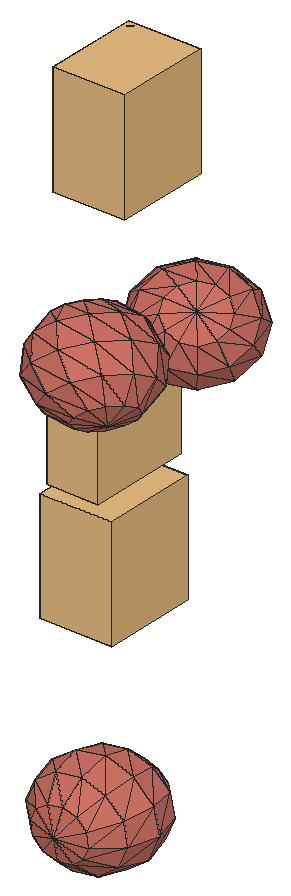
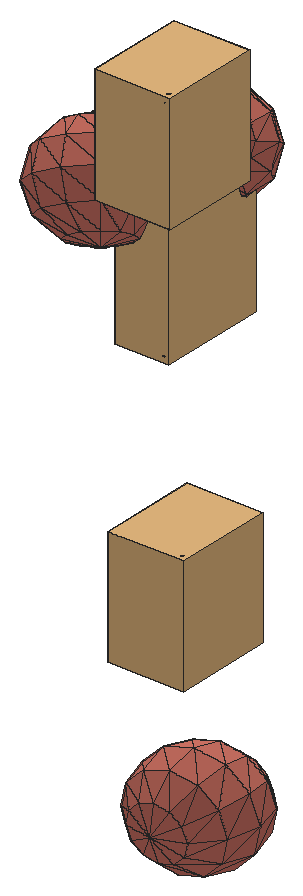
# SketchUp Ruby script. Lengths in inches.
U = 1.inch
M = Sketchup.active_model
def pt(a) = Geom::Point3d.new(a.map { |v| v * U })
def face(e, loops, mat)
  f = e.add_face(loops[0].map { |a| pt(a) })
  loops[1..].each { |l| e.add_face(l.map { |a| pt(a) }).erase! }
  f.material = f.back_material = mat if mat
  f
end
# faces: each face lists its corners as indices into pts; further lists are holes
def faces(e, pts, list, mat = nil) = list.each { |f| face(e, (f[0].is_a?(Array) ? f : [f]).map { |l| l.map { |i| pts[i] } }, mat) }
# xy, xz, yz: faces in a plane at the given z, y or x. An outline is a flat list of corners, or four numbers for a rectangle; further outlines are holes
def ring(l) = l.size == 4 ? [[l[0], l[1]], [l[2], l[1]], [l[2], l[3]], [l[0], l[3]]] : l.each_slice(2).to_a
def flat(e, list, mat, &to3) = list.each { |f| face(e, (f[0].is_a?(Array) ? f : [f]).map { |l| ring(l).map { |u, v| to3.(u, v) } }, mat) }
def xy(e, z, list, mat = nil) = flat(e, list, mat) { |x, y| [x, y, z] }
def xz(e, y, list, mat = nil) = flat(e, list, mat) { |x, z| [x, y, z] }
def yz(e, x, list, mat = nil) = flat(e, list, mat) { |y, z| [x, y, z] }
def lines(e, pts, list) = list.each { |a, b| e.add_line(pt(pts[a]), pt(pts[b])) }
# prism: a flat outline (further loops are holes) pulled along v
def prism(e, loops, v, mat = nil)
  f = face(e, loops, mat); d = Geom::Vector3d.new(v.map { |x| x * U })
  f.pushpull(f.normal.samedirection?(d) ? d.length : -d.length)
end
def box(e, o, s, mat = nil) = prism(e, [[o, [o[0] + s[0], o[1], o[2]], [o[0] + s[0], o[1] + s[1], o[2]], [o[0], o[1] + s[1], o[2]]]], [0, 0, s[2]], mat)
def at(x, y, z, deg = 0) = Geom::Transformation.translation(pt([x, y, z])) * Geom::Transformation.rotation(ORIGIN, Z_AXIS, deg.degrees)
def axes(o, x, y, z) = Geom::Transformation.new([*x, 0, *y, 0, *z, 0, *pt(o).to_a, 1])
def part(name) = M.definitions.add(name)
# library, detail: a bought-in or finely detailed component or shape, given as its bounding box
def library(name, o, s) = part(name).tap { |d| box(d.entities, o, s) }
def detail(e, o, s) = box(e.add_group.entities, o, s)
def put(e, d, t, mat = nil) = e.add_instance(d, t).tap { |i| i.material = mat if mat }
def group(e, t, mat = nil) = e.add_group.tap { |g| g.transformation = t; g.material = mat if mat }.entities
root = M.entities
M.materials.add("green").color = [174, 139, 102]
M.materials.add("vio").color = [206, 114, 100]
c1 = library("3DGeom~144_Defintion",[-424.75,-500,-323.76],[849.5,1000,647.52])
c2 = part("3DGeom~145_Defintion")
p = [[-419.66,479.4,-302.56],[-386.2,481.32,-323.76],[-405.55,478.95,-317.48],[-419.66,479.4,-302.56],[-366.78,485.875,-319.73],[-386.2,481.32,-323.76],
  [-419.66,479.4,-302.56],[-352.51,491.39,-306.47],[-366.78,485.875,-319.73],[-419.66,479.4,-302.56],[-347.21,496.4,-287.52],[-352.51,491.39,-306.47],
  [-419.66,479.4,-302.56],[-424.75,482.55,-283.01],[-419.44,487.56,-264.0625],[-419.66,479.4,-302.56],[-366.41,500,-253.05],[-352.3,499.55,-267.97],
  [-419.66,479.4,-302.56],[-352.3,499.55,-267.97],[-347.21,496.4,-287.52],[-419.66,479.4,-302.56],[-405.17,493.08,-250.79],[-385.76,497.63,-246.76],
  [-419.66,479.4,-302.56],[-385.76,497.63,-246.76],[-366.41,500,-253.05],[-419.66,479.4,-302.56],[-419.44,487.56,-264.0625],[-405.17,493.08,-250.79],
  [368.25,-500,278.25],[381.22,-498.52,262.42],[397.44,-490.86,253.62],[422.57,-466.35,264.06],[368.25,-500,278.25],[397.44,-490.86,253.62],
  [422.57,-466.35,264.06],[397.44,-490.86,253.62],[412.58,-479.09,254.22],[418.52,-450.97,299.13],[368.25,-500,278.25],[422.57,-466.35,264.06],
  [422.57,-466.35,264.06],[424.75,-456.06,280.5],[368.25,-500,278.25],[364.2,-484.62,313.32],[362.02,-494.91,296.88],[364.2,-484.62,313.32],
  [368.25,-500,278.25],[389.33,-460.11,323.76],[389.33,-460.11,323.76],[368.25,-500,278.25],[389.33,-460.11,323.76],[405.55,-452.45,314.97],
  [364.2,-484.62,313.32],[389.33,-460.11,323.76],[374.19,-471.88,323.16]]
faces(c2.entities,p,[[0,1,2],[3,4,5],[6,7,8],[9,10,11],[12,13,14],[15,16,17],[18,19,20],[21,22,23],
  [24,25,26],[27,28,29],[30,31,32],[33,34,35],[36,37,38],[39,40,41],[39,42,43],[44,45,46],
  [47,48,49],[50,51,39],[52,39,53],[54,55,56]],"green")
c3 = library("3DGeom~140_Defintion",[-424.75,-500,-323.76],[849.5,1000,647.52])
c4 = part("3DGeom~141_Defintion")
p = [[-419.66,479.4,-302.56],[-386.2,481.32,-323.76],[-405.55,478.95,-317.48],[-419.66,479.4,-302.56],[-366.78,485.875,-319.73],[-386.2,481.32,-323.76],
  [-419.66,479.4,-302.56],[-352.51,491.39,-306.47],[-366.78,485.875,-319.73],[-419.66,479.4,-302.56],[-347.21,496.4,-287.52],[-352.51,491.39,-306.47],
  [-419.66,479.4,-302.56],[-424.75,482.55,-283.01],[-419.44,487.56,-264.0625],[-419.66,479.4,-302.56],[-366.41,500,-253.05],[-352.3,499.55,-267.97],
  [-419.66,479.4,-302.56],[-352.3,499.55,-267.97],[-347.21,496.4,-287.52],[-419.66,479.4,-302.56],[-405.17,493.08,-250.79],[-385.76,497.63,-246.76],
  [-419.66,479.4,-302.56],[-385.76,497.63,-246.76],[-366.41,500,-253.05],[-419.66,479.4,-302.56],[-419.44,487.56,-264.0625],[-405.17,493.08,-250.79],
  [368.25,-500,278.25],[381.22,-498.52,262.42],[397.44,-490.86,253.62],[422.57,-466.35,264.06],[368.25,-500,278.25],[397.44,-490.86,253.62],
  [422.57,-466.35,264.06],[397.44,-490.86,253.62],[412.58,-479.09,254.22],[418.52,-450.97,299.13],[368.25,-500,278.25],[422.57,-466.35,264.06],
  [422.57,-466.35,264.06],[424.75,-456.06,280.5],[368.25,-500,278.25],[364.2,-484.62,313.32],[362.02,-494.91,296.88],[364.2,-484.62,313.32],
  [368.25,-500,278.25],[389.33,-460.11,323.76],[389.33,-460.11,323.76],[368.25,-500,278.25],[389.33,-460.11,323.76],[405.55,-452.45,314.97],
  [364.2,-484.62,313.32],[389.33,-460.11,323.76],[374.19,-471.88,323.16]]
faces(c4.entities,p,[[0,1,2],[3,4,5],[6,7,8],[9,10,11],[12,13,14],[15,16,17],[18,19,20],[21,22,23],
  [24,25,26],[27,28,29],[30,31,32],[33,34,35],[36,37,38],[39,40,41],[39,42,43],[44,45,46],
  [47,48,49],[50,51,39],[52,39,53],[54,55,56]],"green")
c5 = part("3DGeom~230_Defintion")
p = [[-248.9,29.76,-432.23],[1.27,34.79,-498.32],[1.59,-181.375,-452.05],[251.38,-156.7,-390.8125],[251.1,30.51,-430.88],[-249.48,208.89,-356.66],
  [0.6,241.64,-411.0625],[-249.48,208.89,-356.66],[-248.62,-157.45,-392.16],[1.49,-348.94,-284.65],[251.29,-301.82,-245.84],[-248.62,-157.45,-392.16],
  [-432.38,16.75,-250.32],[-248.62,-157.45,-392.16],[-432.71,120.17,-206.7],[-248.9,29.76,-432.23],[-432.38,16.75,-250.32],[-249.48,208.89,-356.66],
  [-248.9,29.76,-432.23],[433.81,-90.04,-224.86],[433.65,18.05,-247.99],[433.81,-90.04,-224.86],[250.52,209.64,-355.32],[433.65,18.05,-247.99],
  [251.1,30.51,-430.88],[250.52,209.64,-355.32],[-250.19,331.95,-185.71],[-249.48,208.89,-356.66],[-0.22,383.74,-213.67],[250.52,209.64,-355.32],
  [0.6,241.64,-411.0625],[-250.19,331.95,-185.71],[-0.22,383.74,-213.67],[-248.62,-157.45,-392.16],[-248.71,-302.57,-247.1875],[-432.22,-91.34,-227.19],
  [-248.62,-157.45,-392.16],[-248.71,-302.57,-247.1875],[-432.38,16.75,-250.32],[-248.62,-157.45,-392.16],[-432.22,-91.34,-227.19],[251.38,-156.7,-390.8125],
  [433.76,-173.82,-141.16],[251.29,-301.82,-245.84],[251.38,-156.7,-390.8125],[433.81,-90.04,-224.86],[-433.125,191.22,-108],[-250.19,331.95,-185.71],
  [250.52,209.64,-355.32],[433.31,121.47,-204.37],[433.65,18.05,-247.99],[249.81,332.7,-184.37],[250.52,209.64,-355.32],[-0.22,383.74,-213.67],
  [249.81,332.7,-184.37],[250.52,209.64,-355.32],[-248.71,-302.57,-247.1875],[1.49,-348.94,-284.65],[0.99,-423.01,-40.98],[1.49,-348.94,-284.65],
  [250.86,-365.97,-34.82],[1.49,-348.94,-284.65],[251.29,-301.82,-245.84],[-500,-0.75,-1.35],[433.65,18.05,-247.99],[500,0.75,1.35],
  [433.65,18.05,-247.99],[-248.71,-302.57,-247.1875],[-249.14,-366.71,-36.17],[-432.27,-175.12,-143.49],[-249.14,-366.71,-36.17],[251.29,-301.82,-245.84],
  [433.51,-210.86,-19.33],[250.86,-365.97,-34.82],[251.29,-301.82,-245.84],[-250.86,365.97,34.82],[-0.22,383.74,-213.67],[-250.19,331.95,-185.71],
  [-0.99,423.01,40.98],[-0.22,383.74,-213.67],[-250.86,365.97,34.82],[-0.22,383.74,-213.67],[432.9,192.52,-105.67],[249.81,332.7,-184.37],
  [-433.51,210.86,19.33],[-250.86,365.97,34.82],[249.14,366.71,36.17],[249.81,332.7,-184.37],[249.14,366.71,36.17],[-432.52,-212.16,-21.66],
  [432.52,212.16,21.66],[249.14,366.71,36.17],[-249.14,-366.71,-36.17],[0.22,-383.74,213.67],[250.19,-331.95,185.71],[250.19,-331.95,185.71],
  [-249.14,-366.71,-36.17],[-249.81,-332.7,184.37],[-249.81,-332.7,184.37],[250.86,-365.97,-34.82],[433.125,-191.22,108],[250.19,-331.95,185.71],
  [250.86,-365.97,-34.82],[-432.9,-192.52,105.67],[-433.3125,-121.47,204.37],[-433.65,-18.05,247.99],[-433.81,90.04,224.86],[-433.76,173.82,141.16],
  [432.71,-120.17,206.7],[432.38,-16.75,250.32],[432.22,91.34,227.19],[432.38,-16.75,250.32],[432.27,175.12,143.49],[248.71,302.57,247.1875],
  [248.71,302.57,247.1875],[249.14,366.71,36.17],[-251.29,301.82,245.84],[-251.29,301.82,245.84],[-250.86,365.97,34.82],[-1.49,348.94,284.65],
  [248.71,302.57,247.1875],[-251.29,301.82,245.84],[-250.52,-209.64,355.32],[250.19,-331.95,185.71],[248.62,157.45,392.16],[248.62,157.45,392.16],
  [248.71,302.57,247.1875],[-249.81,-332.7,184.37],[-0.6,-241.64,411.0625],[-249.81,-332.7,184.37],[-0.6,-241.64,411.0625],[-250.52,-209.64,355.32],
  [0.22,-383.74,213.67],[250.19,-331.95,185.71],[249.48,-208.89,356.66],[250.19,-331.95,185.71],[249.48,-208.89,356.66],[-251.1,-30.51,430.88],
  [-251.1,-30.51,430.88],[249.48,-208.89,356.66],[432.38,-16.75,250.32],[0.22,-383.74,213.67],[-0.6,-241.64,411.0625],[-433.65,-18.05,247.99],
  [-251.38,156.7,390.8125],[-433.81,90.04,224.86],[-251.38,156.7,390.8125],[248.9,-29.76,432.23],[432.22,91.34,227.19],[248.62,157.45,392.16],
  [432.38,-16.75,250.32],[432.22,91.34,227.19],[-251.38,156.7,390.8125],[-1.49,348.94,284.65],[-251.29,301.82,245.84],[-1.59,181.375,452.05],
  [248.71,302.57,247.1875],[248.71,302.57,247.1875],[-1.49,348.94,284.65],[-433.65,-18.05,247.99],[-251.1,-30.51,430.88],[-251.38,156.7,390.8125],
  [249.48,-208.89,356.66],[432.38,-16.75,250.32],[248.9,-29.76,432.23],[-251.38,156.7,390.8125],[-1.49,348.94,284.65],[-250.52,-209.64,355.32],
  [-1.27,-34.79,498.32],[-250.52,-209.64,355.32],[-251.38,156.7,390.8125]]
faces(c5.entities,p,[[0,1,2],[1,3,2],[1,4,3],[5,1,0],[6,4,1],[7,6,1],[8,2,9],[2,10,9],
  [2,3,10],[0,2,11],[12,0,13],[14,15,16],[14,17,18],[4,19,3],[4,20,21],[22,23,24],
  [6,25,4],[26,6,27],[28,29,30],[31,32,6],[33,9,34],[35,36,37],[38,39,40],[41,42,43],
  [44,45,42],[46,17,14],[46,47,17],[48,49,50],[51,49,52],[53,54,55],[56,57,58],[59,60,58],
  [61,62,60],[16,35,63],[14,16,63],[45,64,65],[66,49,65],[67,58,68],[69,37,70],[35,37,69],
  [71,72,73],[74,42,72],[35,69,63],[42,45,65],[75,76,77],[78,54,79],[80,78,81],[46,14,63],
  [49,82,65],[83,82,49],[84,47,46],[84,85,47],[86,82,87],[78,88,54],[69,70,89],[69,89,63],
  [72,42,65],[84,46,63],[82,90,65],[91,90,82],[92,58,93],[58,94,93],[58,60,95],[96,93,97],
  [89,70,98],[99,100,101],[102,72,100],[89,98,103],[89,103,63],[100,72,65],[103,104,63],[104,105,63],
  [105,106,63],[107,84,63],[106,107,63],[108,100,65],[109,108,65],[110,111,65],[112,110,65],[90,112,65],
  [107,85,84],[113,112,90],[114,90,115],[107,116,85],[117,78,118],[119,120,88],[119,88,78],[121,119,78],
  [103,98,122],[103,122,104],[123,100,108],[106,116,107],[124,110,112],[125,112,126],[127,93,128],[129,130,131],
  [132,133,134],[135,108,136],[104,122,137],[104,138,105],[139,108,140],[141,134,142],[143,144,145],[106,146,116],
  [147,148,149],[147,150,151],[152,153,154],[155,149,156],[155,157,158],[159,160,161],[162,163,164],[165,155,166],
  [167,142,168],[169,168,160],[142,134,147],[160,155,170],[168,149,155],[168,147,149],[142,147,168],[160,168,155]],"vio")
c6 = library("3DGeom~152_Defintion",[-440.97,-500,-219.08],[881.94,1000,438.17])
c7 = part("3DGeom~153_Defintion")
p = [[-380.69,-485.53,-210.54],[-411.26,-467,-218.1875],[-394.16,-475.51,-219.08],[-380.69,-485.53,-210.54],[-434.74,-476.74,-157.14],[-411.26,-467,-218.1875],
  [-438.29,-462.61,-191.49],[-411.26,-467,-218.1875],[-438.29,-462.61,-191.49],[-427.41,-462.28,-208.09],[-377.14,-499.67,-176.1875],[-434.74,-476.74,-157.14],
  [-380.69,-485.53,-210.54],[-377.14,-499.67,-176.1875],[-380.69,-485.53,-210.54],[-374.46,-494.375,-194.84],[-434.74,-476.74,-157.14],[-440.97,-467.9,-172.84],
  [-438.29,-462.61,-191.49],[-404.17,-495.28,-149.49],[-377.14,-499.67,-176.1875],[-388.02,-500,-159.59],[-404.17,-495.28,-149.49],[-434.74,-476.74,-157.14],
  [-404.17,-495.28,-149.49],[-421.27,-486.76,-148.59],[402.51,492.03,208.37],[431.04,458.58,149.1],[419.28,470.25,140.95],[402.51,492.03,208.37],
  [419.28,470.25,140.95],[406.85,483.28,142.92],[402.51,492.03,208.37],[406.85,483.28,142.92],[397.08,494.16,154.49],[402.51,492.03,208.37],
  [438.98,451.39,165.19],[431.04,458.58,149.1],[402.51,492.03,208.37],[397.08,494.16,154.49],[392.58,500,172.55],[402.51,492.03,208.37],
  [440.97,450.61,184.92],[438.98,451.39,165.19],[402.51,492.03,208.37],[392.58,500,172.55],[394.57,499.22,192.28],[402.51,492.03,208.37],
  [436.48,456.44,202.98],[440.97,450.61,184.92],[402.51,492.03,208.37],[426.7,467.33,214.55],[402.51,492.03,208.37],[414.27,480.36,216.53],
  [426.7,467.33,214.55]]
faces(c7.entities,p,[[0,1,2],[3,4,5],[5,4,6],[7,8,9],[10,11,12],[13,14,15],[16,17,18],[19,20,21],
  [22,11,10],[23,24,25],[26,27,28],[29,30,31],[32,33,34],[35,36,37],[38,39,40],[41,42,43],
  [44,45,46],[47,48,49],[50,51,48],[52,53,54]],"green")
c8 = part("3DGeom~238_Defintion")
p = [[47.04,-55.62,-493.71],[-13.56,-317.59,-331.8],[-140.27,-151.99,-445.55],[202.73,-206.32,-387.4],[187.3,88.625,-451.96],[-121.25,109.98,-467.72],
  [-40.27,193.26,-443.62],[-229.4,54.34,-439.92],[-257.06,246.11,-316.41],[364.69,-39.76,-339.2],[242.94,242.1,-331.5],[-8.15,281.87,-374.07],
  [-226.21,-343.77,-187.29],[-324.43,-174.66,-320.41],[-335.72,41.26,-367.67],[202.73,-206.32,-387.4],[116.79,-398.1,-129.14],[-13.56,-317.59,-331.8],
  [202.73,-206.32,-387.4],[304.09,-301.73,-177.3],[364.69,-39.76,-339.2],[304.09,-301.73,-177.3],[202.73,-206.32,-387.4],[-33.49,352.06,-277.72],
  [242.94,242.1,-331.5],[-8.15,281.87,-374.07],[-33.49,352.06,-277.72],[-335.72,41.26,-367.67],[-324.43,-174.66,-320.41],[-456.1,-117.55,-151.8],
  [-335.72,41.26,-367.67],[-411.74,74.22,-270.32],[-335.72,41.26,-367.67],[-257.06,246.11,-316.41],[364.69,-39.76,-339.2],[444.36,-157.49,-135.55],
  [304.09,-301.73,-177.3],[428.9375,137.45,-200.11],[364.69,-39.76,-339.2],[428.9375,137.45,-200.11],[-13.56,-317.59,-331.8],[-67.38,-420.77,-4],
  [-226.21,-343.77,-187.29],[-13.56,-317.59,-331.8],[199.05,363.67,-164.61],[428.9375,137.45,-200.11],[242.94,242.1,-331.5],[-33.49,352.06,-277.72],
  [199.05,363.67,-164.61],[242.94,242.1,-331.5],[-324.43,-174.66,-320.41],[-226.21,-343.77,-187.29],[-378.25,-277.83,7.4],[-324.43,-174.66,-320.41],
  [-437.09,144.42,-173.96],[-257.06,246.11,-316.41],[-404.96,233.02,-104.42],[-257.06,246.11,-316.41],[-323.98,316.3,-80.32],[-257.06,246.11,-316.41],
  [-323.98,316.3,-80.32],[-215.84,371.9375,-108.12],[-257.06,246.11,-316.41],[-109.51,385.02,-180.37],[-33.49,352.06,-277.72],[-257.06,246.11,-316.41],
  [-257.06,246.11,-316.41],[-33.49,352.06,-277.72],[-500,4.02,15.09],[428.9375,137.45,-200.11],[500,-4.02,-15.09],[378.25,277.83,-7.4],
  [428.9375,137.45,-200.11],[199.05,363.67,-164.61],[428.9375,137.45,-200.11],[-226.21,-343.77,-187.29],[-199.05,-363.67,164.61],[-226.21,-343.77,-187.29],
  [-199.05,-363.67,164.61],[-378.25,-277.83,7.4],[67.38,420.77,4],[215.84,-371.9375,108.12],[323.98,-316.3,80.32],[323.98,-316.3,80.32],
  [304.09,-301.73,-177.3],[-444.36,157.49,135.55],[378.25,277.83,-7.4],[-428.9375,-137.45,200.11],[404.96,-233.02,104.42],[323.98,-316.3,80.32],
  [109.51,-385.02,180.37],[-116.78,398.1,129.14],[-304.09,301.73,177.3],[-304.09,301.73,177.3],[-323.98,316.3,-80.32],[-304.09,301.73,177.3],
  [437.09,-144.42,173.96],[456.1,117.55,151.8],[226.21,343.77,187.29],[226.21,343.77,187.29],[378.25,277.83,-7.4],[33.49,-352.06,277.72],
  [-199.05,-363.67,164.61],[-199.05,-363.67,164.61],[-242.94,-242.09,331.5],[-242.94,-242.09,331.5],[-364.69,39.76,339.2],[257.06,-246.11,316.41],
  [323.98,-316.3,80.32],[257.06,-246.11,316.41],[257.06,-246.11,316.41],[13.56,317.59,331.8],[-202.73,206.32,387.4],[-202.73,206.32,387.4],
  [-304.09,301.73,177.3],[411.74,-74.22,270.32],[324.43,174.66,320.41],[226.21,343.77,187.29],[-199.05,-363.67,164.61],[8.15,-281.87,374.07],
  [-242.94,-242.09,331.5],[-199.05,-363.67,164.61],[8.15,-281.87,374.07],[257.06,-246.11,316.41],[-202.73,206.32,387.4],[13.56,317.59,331.8],
  [324.43,174.66,320.41],[226.21,343.77,187.29],[-428.9375,-137.45,200.11],[-242.94,-242.09,331.5],[-187.3,-88.625,451.96],[-428.9375,-137.45,200.11],
  [-364.69,39.76,339.2],[335.72,-41.26,367.67],[257.06,-246.11,316.41],[8.15,-281.87,374.07],[33.49,-352.06,277.72],[257.06,-246.11,316.41],
  [40.27,-193.26,443.62],[257.06,-246.11,316.41],[121.25,-109.98,467.72],[257.06,-246.11,316.41],[229.4,-54.34,439.92],[257.06,-246.11,316.41],
  [335.72,-41.26,367.67],[257.06,-246.11,316.41],[140.27,151.99,445.55],[335.72,-41.26,367.67],[324.43,174.66,320.41],[13.56,317.59,331.8],
  [324.43,174.66,320.41],[-202.73,206.32,387.4],[13.56,317.59,331.8],[-364.69,39.76,339.2],[-47.04,55.62,493.71],[-364.69,39.76,339.2],
  [-202.73,206.32,387.4],[335.72,-41.26,367.67],[-202.73,206.32,387.4]]
faces(c8.entities,p,[[0,1,2],[0,3,1],[4,3,0],[5,0,2],[6,0,5],[6,4,0],[5,2,7],[5,7,8],
  [6,5,8],[4,9,3],[10,9,4],[11,4,6],[11,10,4],[2,12,13],[2,1,12],[7,2,13],
  [11,6,8],[7,13,14],[7,14,8],[15,16,17],[18,19,16],[20,21,22],[23,24,25],[26,11,8],
  [27,28,29],[30,29,31],[32,31,33],[34,35,36],[37,35,38],[10,39,9],[40,41,42],[43,16,41],
  [44,45,46],[47,48,49],[50,51,52],[53,52,29],[31,54,55],[54,56,57],[56,58,59],[60,61,62],
  [63,64,65],[61,63,66],[63,48,67],[31,29,68],[31,68,54],[69,70,35],[71,70,72],[73,71,74],
  [75,41,76],[77,78,79],[63,80,48],[61,80,63],[19,81,16],[19,82,81],[35,83,84],[54,68,85],
  [54,85,56],[80,86,48],[29,52,87],[29,87,68],[35,88,89],[70,88,35],[16,90,41],[16,81,90],
  [60,91,61],[61,91,80],[56,85,92],[56,93,94],[60,95,91],[70,96,88],[97,96,70],[71,97,70],
  [98,97,71],[80,99,100],[41,101,102],[41,90,101],[91,99,80],[52,103,104],[52,105,87],[68,87,106],
  [68,106,85],[81,82,107],[108,88,109],[88,96,110],[90,81,107],[95,111,91],[91,111,99],[85,106,112],
  [85,113,114],[97,115,96],[116,115,97],[117,116,97],[118,119,120],[121,101,122],[96,115,123],[95,124,111],
  [101,90,107],[125,126,127],[128,129,130],[131,130,132],[115,133,134],[116,133,115],[135,136,137],[138,135,139],
  [140,138,141],[142,140,143],[144,142,145],[146,147,148],[149,146,150],[129,135,138],[129,138,130],[151,146,152],
  [153,130,154],[155,154,156],[146,142,157],[158,154,146],[154,140,142],[154,142,146],[130,138,140],[130,140,154]],"vio")
c9 = part("3DGeom~206_Defintion")
p = [[-12.5,-12.78,-500],[-167.87,-176.1875,-423.23],[-275,-119.8,-393.5],[139.12,-146.19,-448.74],[321.29,0,-383.61],[-198.05,84.89,-448.51],
  [146.22,154.06,-442.79],[216.18,-279.61,-308.47],[-80.33,-253.22,-393.64],[410.28,-154.06,-221.63],[410.28,-154.06,-221.63],[-373.01,-99.16,-312.41],
  [-373.01,-99.16,-312.41],[-367.81,120.64,-308.0625],[-68.03,266.84,-383.34],[-367.81,120.64,-308.0625],[-68.03,266.84,-383.34],[417.375,146.19,-215.68],
  [417.375,146.19,-215.68],[265.76,279.61,-266.94],[265.76,279.61,-266.94],[-68.03,266.84,-383.34],[-278.26,-292.39,-233.06],[-278.26,-292.39,-233.06],
  [-35.84,-330.25,-312.65],[-278.26,-292.39,-233.06],[-373.01,-99.16,-312.41],[-275,-119.8,-393.5],[-278.26,-292.39,-233.06],[494.4375,12.78,-75.41],
  [410.28,-154.06,-221.63],[321.29,0,-383.61],[321.29,0,-383.61],[417.375,146.19,-215.68],[-68.03,266.84,-383.34],[-367.81,120.64,-308.0625],
  [-264.06,308.11,-221.16],[80.21,377.28,-215.45],[-68.03,266.84,-383.34],[-264.06,308.11,-221.16],[265.76,279.61,-266.94],[-68.03,266.84,-383.34],
  [80.21,377.28,-215.45],[-35.84,-330.25,-312.65],[-46.32,-386.64,-201.97],[-278.26,-292.39,-233.06],[198.04,-377.28,-116.76],[-35.84,-330.25,-312.65],
  [198.04,-377.28,-116.76],[-35.84,-330.25,-312.65],[216.18,-279.61,-308.47],[-435.64,-119.8,-201.7],[-278.26,-292.39,-233.06],[-367.81,120.64,-308.0625],
  [389.33,-266.84,-0.27],[198.04,-377.28,-116.76],[216.18,-279.61,-308.47],[216.18,-279.61,-308.47],[-476.3,84.89,-116.29],[-264.06,308.11,-221.16],
  [401.625,253.22,10.03],[265.76,279.61,-266.94],[265.76,279.61,-266.94],[314.09,330.25,-19.5625],[314.09,330.25,-19.5625],[265.76,279.61,-266.94],
  [-108.95,-407.27,-91.25],[-206.96,-386.64,-10.17],[-314.09,-330.25,19.5625],[-314.09,-330.25,19.5625],[-401.625,-253.22,-10.03],[-278.26,-292.39,-233.06],
  [-446.12,-176.1875,-91.02],[-278.26,-292.39,-233.06],[-278.26,-292.39,-233.06],[476.3,-84.89,116.29],[-264.06,308.11,-221.16],[-389.33,266.84,0.27],
  [-89.55,413.03,-75],[-389.33,266.84,0.27],[446.12,176.1875,91.02],[206.96,386.64,10.17],[89.55,-413.03,75],[198.04,-377.28,-116.76],
  [264.06,-308.11,221.16],[198.04,-377.28,-116.76],[264.06,-308.11,221.16],[198.04,-377.28,-116.76],[389.33,-266.84,-0.27],[-494.4375,-12.78,75.41],
  [-80.21,-377.28,215.45],[435.64,119.8,201.7],[-389.33,266.84,0.27],[-198.04,377.28,116.76],[108.95,407.27,91.25],[314.09,330.25,-19.5625],
  [278.26,292.39,233.06],[278.26,292.39,233.06],[-265.76,-279.61,266.94],[-265.76,-279.61,266.94],[-417.375,-146.19,215.68],[-314.09,-330.25,19.5625],
  [-417.375,-146.19,215.68],[367.81,-120.64,308.0625],[264.06,-308.11,221.16],[367.81,-120.64,308.0625],[-410.28,154.06,221.63],[-198.04,377.28,116.76],
  [-410.28,154.06,221.63],[278.26,292.39,233.06],[-417.375,-146.19,215.68],[-314.09,-330.25,19.5625],[-265.76,-279.61,266.94],[68.03,-266.84,383.34],
  [68.03,-266.84,383.34],[264.06,-308.11,221.16],[-410.28,154.06,221.63],[-417.375,-146.19,215.68],[46.32,386.64,201.97],[278.26,292.39,233.06],
  [373.01,99.16,312.41],[367.81,-120.64,308.0625],[-198.04,377.28,116.76],[-410.28,154.06,221.63],[-216.18,279.61,308.47],[-216.18,279.61,308.47],
  [-216.18,279.61,308.47],[35.84,330.25,312.65],[35.84,330.25,312.65],[278.26,292.39,233.06],[-146.22,-154.06,442.79],[-265.76,-279.61,266.94],
  [-80.21,-377.28,215.45],[-80.21,-377.28,215.45],[68.03,-266.84,383.34],[-321.29,0,383.61],[-417.375,-146.19,215.68],[-410.28,154.06,221.63],
  [-417.375,-146.19,215.68],[-321.29,0,383.61],[198.05,-84.89,448.51],[264.06,-308.11,221.16],[367.81,-120.64,308.0625],[-216.18,279.61,308.47],
  [-410.28,154.06,221.63],[275,119.8,393.5],[167.87,176.1875,423.23],[275,119.8,393.5],[278.26,292.39,233.06],[80.33,253.22,393.64],
  [278.26,292.39,233.06],[35.84,330.25,312.65],[278.26,292.39,233.06],[275,119.8,393.5],[275,119.8,393.5],[373.01,99.16,312.41],
  [-139.12,146.19,448.74],[12.5,12.78,500],[275,119.8,393.5]]
faces(c9.entities,p,[[0,1,2],[3,1,0],[4,3,0],[0,2,5],[6,0,5],[4,0,6],[7,8,3],[9,7,3],
  [3,8,1],[10,3,4],[5,2,11],[5,12,13],[14,5,15],[6,5,16],[17,4,6],[18,6,19],
  [20,6,21],[2,1,22],[1,8,23],[8,24,25],[7,24,8],[26,27,28],[29,30,31],[29,32,33],
  [34,35,36],[37,38,39],[40,41,42],[43,44,45],[46,44,47],[48,49,50],[51,26,52],[53,26,51],
  [54,55,56],[54,57,30],[53,51,58],[59,53,58],[60,33,61],[60,62,63],[64,65,37],[66,67,45],
  [44,66,45],[67,68,45],[69,70,71],[70,72,73],[72,51,74],[75,54,30],[75,30,29],[76,58,77],
  [78,39,79],[37,39,78],[80,29,33],[80,33,60],[64,37,81],[81,37,78],[82,66,44],[82,44,83],
  [58,51,72],[84,82,85],[86,87,88],[58,72,89],[77,58,89],[90,66,82],[90,67,66],[89,72,70],
  [91,75,29],[91,29,80],[78,92,93],[94,78,93],[81,78,94],[60,95,96],[64,81,97],[98,68,67],
  [99,67,90],[100,70,101],[89,70,102],[103,104,54],[105,54,75],[77,89,106],[107,77,108],[80,60,96],
  [81,94,109],[110,111,112],[113,90,82],[114,82,115],[116,89,117],[91,80,96],[94,118,119],[94,93,118],
  [120,121,75],[120,75,91],[122,123,124],[118,93,125],[120,91,96],[118,126,127],[118,128,129],[130,131,132],
  [130,133,134],[135,136,131],[137,138,139],[140,134,141],[140,141,142],[143,144,135],[145,120,96],[146,147,148],
  [149,146,150],[151,149,152],[135,131,130],[153,140,142],[154,142,155],[143,135,156],[151,143,156],[151,156,149],
  [157,130,134],[157,134,140],[156,135,130],[146,140,158],[149,156,157],[149,157,146],[146,157,140],[156,130,157]],"vio")
g1 = group(root,at(15.3125,38.42,26.21))
put(g1,c1,axes([-1.98,0.73,11.8125],[0,0.00037,0],[0,0,-0.00037],[-0.00037,0,0]),"green")
put(g1,c2,axes([-1.98,0.73,11.8125],[0,0.00037,0],[0,0,-0.00037],[-0.00037,0,0]),"green")
g2 = group(root,at(15.3125,38.42,26.21))
put(g2,c3,axes([-1.93,0.72,13.1],[0,0.00037,0],[0,0,-0.00037],[-0.00037,0,0]),"green")
put(g2,c4,axes([-1.93,0.72,13.1],[0,0.00037,0],[0,0,-0.00037],[-0.00037,0,0]),"green")
g3 = group(root,at(15.3125,38.42,26.21))
put(g3,c5,axes([-1.92,0.6,11.11],[0,0.00039,0],[0,0,-0.00039],[-0.00039,0,0]),"vio")
g4 = group(root,at(15.3125,38.42,26.21))
put(g4,c6,axes([-1.7,0.38,12.49],[0,0.00039,0],[0,0,-0.00039],[-0.00039,0,0]),"green")
put(g4,c7,axes([-1.7,0.38,12.49],[0,0.00039,0],[0,0,-0.00039],[-0.00039,0,0]),"green")
g5 = group(root,at(15.3125,38.42,26.21))
put(g5,c8,axes([-1.62,0.2,12.71],[0,0.00039,0],[0,0,-0.00039],[-0.00039,0,0]),"vio")
g6 = group(root,at(15.3125,38.42,26.21))
put(g6,c9,axes([-1.54,0.52,12.72],[0,0.00039,0],[0,0,-0.00039],[-0.00039,0,0]),"vio")
